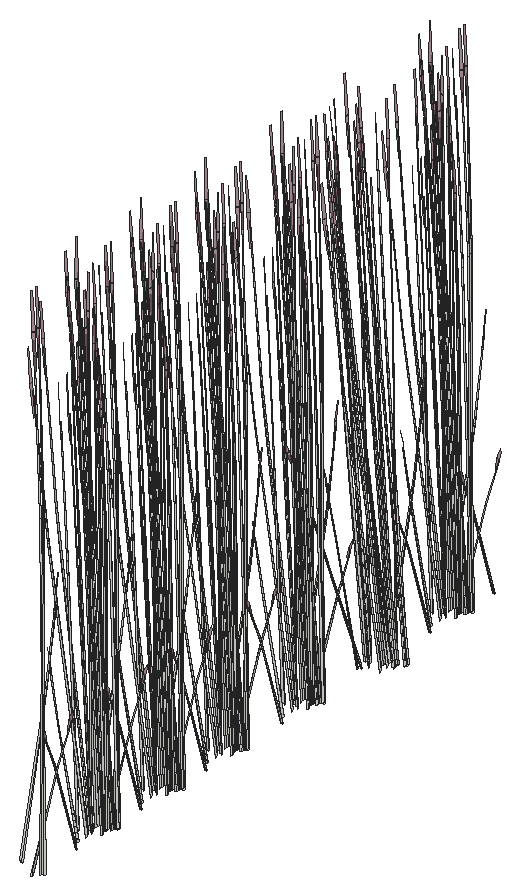
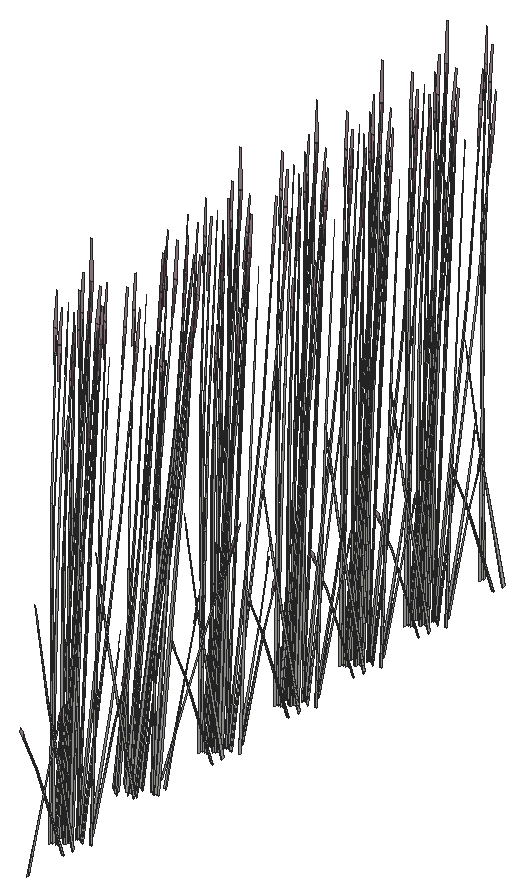
# SketchUp Ruby script. Lengths in inches.
U = 1.inch
M = Sketchup.active_model
def pt(a) = Geom::Point3d.new(a.map { |v| v * U })
def face(e, loops, mat)
  f = e.add_face(loops[0].map { |a| pt(a) })
  loops[1..].each { |l| e.add_face(l.map { |a| pt(a) }).erase! }
  f.material = f.back_material = mat if mat
  f
end
# faces: each face lists its corners as indices into pts; further lists are holes
def faces(e, pts, list, mat = nil) = list.each { |f| face(e, (f[0].is_a?(Array) ? f : [f]).map { |l| l.map { |i| pts[i] } }, mat) }
# xy, xz, yz: faces in a plane at the given z, y or x. An outline is a flat list of corners, or four numbers for a rectangle; further outlines are holes
def ring(l) = l.size == 4 ? [[l[0], l[1]], [l[2], l[1]], [l[2], l[3]], [l[0], l[3]]] : l.each_slice(2).to_a
def flat(e, list, mat, &to3) = list.each { |f| face(e, (f[0].is_a?(Array) ? f : [f]).map { |l| ring(l).map { |u, v| to3.(u, v) } }, mat) }
def xy(e, z, list, mat = nil) = flat(e, list, mat) { |x, y| [x, y, z] }
def xz(e, y, list, mat = nil) = flat(e, list, mat) { |x, z| [x, y, z] }
def yz(e, x, list, mat = nil) = flat(e, list, mat) { |y, z| [x, y, z] }
def lines(e, pts, list) = list.each { |a, b| e.add_line(pt(pts[a]), pt(pts[b])) }
# prism: a flat outline (further loops are holes) pulled along v
def prism(e, loops, v, mat = nil)
  f = face(e, loops, mat); d = Geom::Vector3d.new(v.map { |x| x * U })
  f.pushpull(f.normal.samedirection?(d) ? d.length : -d.length)
end
def box(e, o, s, mat = nil) = prism(e, [[o, [o[0] + s[0], o[1], o[2]], [o[0] + s[0], o[1] + s[1], o[2]], [o[0], o[1] + s[1], o[2]]]], [0, 0, s[2]], mat)
def at(x, y, z, deg = 0) = Geom::Transformation.translation(pt([x, y, z])) * Geom::Transformation.rotation(ORIGIN, Z_AXIS, deg.degrees)
def axes(o, x, y, z) = Geom::Transformation.new([*x, 0, *y, 0, *z, 0, *pt(o).to_a, 1])
def part(name) = M.definitions.add(name)
# library, detail: a bought-in or finely detailed component or shape, given as its bounding box
def library(name, o, s) = part(name).tap { |d| box(d.entities, o, s) }
def detail(e, o, s) = box(e.add_group.entities, o, s)
def put(e, d, t, mat = nil) = e.add_instance(d, t).tap { |i| i.material = mat if mat }
def group(e, t, mat = nil) = e.add_group.tap { |g| g.transformation = t; g.material = mat if mat }.entities
root = M.entities
M.materials.add("LightPink_Translucent").color = [144, 107, 117]
M.materials["LightPink_Translucent"].alpha = 0.75
c1 = part("blade")
p = [[2.15,0.21,22],[0,0.17,0],[0.09,0.45,0],[2.18,0.31,22],[2.29,0.31,22],[0.38,0.45,0],
  [2.48,0.24,33],[2.49,0.24,33],[2.48,0.22,33]]
faces(c1.entities,p,[[0,1,2,3],[4,5,2,3],[6,3,4,7],[8,0,3,6]])
c2 = part("seeds")
p = [[0.3,-0.1,1.38],[-0.01,-0.03,1.59],[-0.01,-0.03,0.03],[0.14,-0.07,-0.07],[0.29,-0.03,3],[0.15,0.01,3.11]]
faces(c2.entities,p,[[0,1,2,3],[1,0,4,5]],"LightPink_Translucent")
c3 = part("blade with seeds")
put(c3.entities,c1,at(0,0,0))
put(c3.entities,c2,axes([2.4,0.25,30.99],[1.5799,-0.05474,1.17369],[-0.12525,1.92788,0.29478],[-0.07173,-0.02425,1.56792]))
put(root,c3,axes([334.62,388.33,50.06],[0.63212,0.12701,0.27176],[-0.15814,0.45398,-0.32244],[-0.10462,0.05682,1.45692]))
put(root,c3,axes([335,388.57,50.1],[0.31568,0.39156,0],[-0.52815,0.21836,-0.456],[-0.12029,0.04973,1.44655]))
put(root,c3,axes([333.34,388.69,49.32],[0.08172,-0.02126,1.55816],[0.49154,0.11703,-0.23804],[0.01437,0.1319,0.26541]))
put(root,c3,axes([332.21,388.75,50.49],[0.45869,-0.0692,0.0575],[0.10545,0.27878,-0.76259],[-0.02908,0.14112,0.68355]))
put(root,c3,axes([333.7,394.53,49.32],[-0.08469,0.01408,1.55816],[-0.46834,-0.15847,-0.23804],[0.00786,-0.13218,0.26541]))
put(root,c3,axes([333,396.42,49.85],[-0.20736,-0.4007,-0.61707],[0.59731,-0.14431,-0.16195],[-0.02292,-0.13569,1.36206]))
put(root,c3,axes([333.61,394.8,49.88],[-0.34892,0.22417,-0.0344],[-0.3197,-0.24551,-0.15595],[-0.02251,-0.06957,0.51438]))
put(root,c3,axes([333.32,396.53,49.95],[0.24498,-0.3521,-0.39531],[0.50902,0.16945,0.19025],[0,-0.08116,1.26923]))
put(root,c3,axes([332.02,396.375,49.79],[0.35245,-0.2438,-0.27372],[0.35245,0.2438,0.27372],[0,-0.07853,1.22797]))
put(root,c3,axes([333.25,396.82,50.36],[-0.56863,-0.18645,-0.25709],[0.2738,-0.39352,-0.44182],[-0.01787,-0.09662,1.41118]))
put(root,c3,axes([333.42,396.58,50.09],[0.21952,0.43694,0.40429],[-0.62724,0.15194,0.15865],[0.00767,-0.08029,1.40366]))
put(root,c3,axes([333.31,396.93,50.4],[-0.24498,0.3521,0.39531],[-0.50902,-0.16945,-0.19025],[0,-0.08116,1.26923]))
put(root,c3,axes([334.36,396.97,50.03],[-0.46965,-0.33633,-0.05417],[0.46994,-0.33653,0],[-0.0164,-0.01174,1.55135]))
put(root,c3,axes([333.47,397.01,50.09],[0.63817,0.08233,0.40429],[-0.12987,0.46497,0.15865],[-0.09326,-0.0449,1.40366]))
put(root,c3,axes([333.13,397.75,50.1875],[0.54257,-0.10371,0.15589],[0.13397,0.38597,0.31002],[-0.04839,-0.05624,1.41735]))
put(root,c3,axes([333.94,397.66,49.95],[-0.16474,-0.33688,0],[0.47043,-0.11798,0],[0,0,1.36402]))
put(root,c3,axes([334.74,397.77,50.1875],[0.14586,-0.38834,0.15589],[0.53375,0.1099,0.31002],[-0.0922,0.00189,1.41735]))
put(root,c3,axes([333.83,397.82,49.94],[-0.50902,-0.17543,0],[0.24498,-0.36452,0],[0,0,1.43768]))
put(root,c3,axes([334.49,397.09,50.4],[0.54829,-0.02412,0.39531],[0.04958,0.40041,-0.19025],[-0.09816,0.04058,1.26923]))
put(root,c3,axes([334.61,398.21,49.9375],[-0.31175,-0.39292,-0.04544],[0.52815,-0.21836,0.456],[-0.13015,0.03741,1.44584]))
put(root,c3,axes([334.5,397.26,50.3125],[0.37303,0.23477,0.12794],[-0.31115,0.26487,-0.36534],[-0.08661,0.03581,1.11991]))
put(root,c3,axes([334.89,397.98,50.19],[0.47255,-0.19538,0.43871],[0.28245,0.35034,0],[-0.10763,0.0445,1.3917]))
put(root,c3,axes([334.46,398.16,49.79],[-0.47106,-0.09668,-0.27372],[0.11861,-0.34048,0.27372],[-0.09497,0.03926,1.22797]))
put(root,c3,axes([334.38,397.17,50.36],[0.05884,0.44587,-0.25709],[-0.6128,0.02696,-0.44182],[-0.10791,0.05939,1.41118]))
put(root,c3,axes([334.62,398.01,50.06],[0.63212,0.12701,0.27176],[-0.15814,0.45398,-0.32244],[-0.10462,0.05682,1.45692]))
put(root,c3,axes([335,398.25,50.1],[0.31568,0.39156,0],[-0.52815,0.21836,-0.456],[-0.12029,0.04973,1.44655]))
put(root,c3,axes([333.7,402.99,49.32],[-0.08469,0.01408,1.55816],[-0.46834,-0.15847,-0.23804],[0.00786,-0.13218,0.26541]))
put(root,c3,axes([333.34,398.375,49.32],[0.08172,-0.02126,1.55816],[0.49154,0.11703,-0.23804],[0.01437,0.1319,0.26541]))
put(root,c3,axes([332.21,398.43,50.49],[0.45869,-0.0692,0.0575],[0.10545,0.27878,-0.76259],[-0.02908,0.14112,0.68355]))
put(root,c3,axes([333,404.89,49.85],[-0.20736,-0.4007,-0.61707],[0.59731,-0.14431,-0.16195],[-0.02292,-0.13569,1.36206]))
put(root,c3,axes([333.61,403.26,49.88],[-0.34892,0.22417,-0.0344],[-0.3197,-0.24551,-0.15595],[-0.02251,-0.06957,0.51438]))
put(root,c3,axes([333.32,404.99,49.95],[0.24498,-0.3521,-0.39531],[0.50902,0.16945,0.19025],[0,-0.08116,1.26923]))
put(root,c3,axes([332.02,404.84,49.79],[0.35245,-0.2438,-0.27372],[0.35245,0.2438,0.27372],[0,-0.07853,1.22797]))
put(root,c3,axes([333.25,405.28,50.36],[-0.56863,-0.18645,-0.25709],[0.2738,-0.39352,-0.44182],[-0.01787,-0.09662,1.41118]))
put(root,c3,axes([333.42,405.04,50.09],[0.21952,0.43694,0.40429],[-0.62724,0.15194,0.15865],[0.00767,-0.08029,1.40366]))
put(root,c3,axes([333.31,405.39,50.4],[-0.24498,0.3521,0.39531],[-0.50902,-0.16945,-0.19025],[0,-0.08116,1.26923]))
put(root,c3,axes([334.36,405.43,50.03],[-0.46965,-0.33633,-0.05417],[0.46994,-0.33653,0],[-0.0164,-0.01174,1.55135]))
put(root,c3,axes([333.47,405.47,50.09],[0.63817,0.08233,0.40429],[-0.12987,0.46497,0.15865],[-0.09326,-0.0449,1.40366]))
put(root,c3,axes([333.13,406.21,50.1875],[0.54257,-0.10371,0.15589],[0.13397,0.38597,0.31002],[-0.04839,-0.05624,1.41735]))
put(root,c3,axes([333.94,406.125,49.95],[-0.16474,-0.33688,0],[0.47043,-0.11798,0],[0,0,1.36402]))
put(root,c3,axes([334.74,406.24,50.1875],[0.14586,-0.38834,0.15589],[0.53375,0.1099,0.31002],[-0.0922,0.00189,1.41735]))
put(root,c3,axes([333.83,406.28,49.94],[-0.50902,-0.17543,0],[0.24498,-0.36452,0],[0,0,1.43768]))
put(root,c3,axes([334.49,405.55,50.4],[0.54829,-0.02412,0.39531],[0.04958,0.40041,-0.19025],[-0.09816,0.04058,1.26923]))
put(root,c3,axes([334.61,406.67,49.9375],[-0.31175,-0.39292,-0.04544],[0.52815,-0.21836,0.456],[-0.13015,0.03741,1.44584]))
put(root,c3,axes([334.5,405.72,50.3125],[0.37303,0.23477,0.12794],[-0.31115,0.26487,-0.36534],[-0.08661,0.03581,1.11991]))
put(root,c3,axes([334.89,406.44,50.19],[0.47255,-0.19538,0.43871],[0.28245,0.35034,0],[-0.10763,0.0445,1.3917]))
put(root,c3,axes([334.46,406.62,49.79],[-0.47106,-0.09668,-0.27372],[0.11861,-0.34048,0.27372],[-0.09497,0.03926,1.22797]))
put(root,c3,axes([334.38,405.63,50.36],[0.05884,0.44587,-0.25709],[-0.6128,0.02696,-0.44182],[-0.10791,0.05939,1.41118]))
put(root,c3,axes([334.62,406.47,50.06],[0.63212,0.12701,0.27176],[-0.15814,0.45398,-0.32244],[-0.10462,0.05682,1.45692]))
put(root,c3,axes([335,406.72,50.1],[0.31568,0.39156,0],[-0.52815,0.21836,-0.456],[-0.12029,0.04973,1.44655]))
put(root,c3,axes([333.7,411.45,49.32],[-0.08469,0.01408,1.55816],[-0.46834,-0.15847,-0.23804],[0.00786,-0.13218,0.26541]))
put(root,c3,axes([333.34,406.83,49.32],[0.08172,-0.02126,1.55816],[0.49154,0.11703,-0.23804],[0.01437,0.1319,0.26541]))
put(root,c3,axes([332.21,406.89,50.49],[0.45869,-0.0692,0.0575],[0.10545,0.27878,-0.76259],[-0.02908,0.14112,0.68355]))
put(root,c3,axes([333,413.35,49.85],[-0.20736,-0.4007,-0.61707],[0.59731,-0.14431,-0.16195],[-0.02292,-0.13569,1.36206]))
put(root,c3,axes([333.61,411.73,49.88],[-0.34892,0.22417,-0.0344],[-0.3197,-0.24551,-0.15595],[-0.02251,-0.06957,0.51438]))
put(root,c3,axes([333.32,413.45,49.95],[0.24498,-0.3521,-0.39531],[0.50902,0.16945,0.19025],[0,-0.08116,1.26923]))
put(root,c3,axes([332.02,413.3,49.79],[0.35245,-0.2438,-0.27372],[0.35245,0.2438,0.27372],[0,-0.07853,1.22797]))
put(root,c3,axes([333.25,413.75,50.36],[-0.56863,-0.18645,-0.25709],[0.2738,-0.39352,-0.44182],[-0.01787,-0.09662,1.41118]))
put(root,c3,axes([333.42,413.51,50.09],[0.21952,0.43694,0.40429],[-0.62724,0.15194,0.15865],[0.00767,-0.08029,1.40366]))
put(root,c3,axes([333.31,413.85,50.4],[-0.24498,0.3521,0.39531],[-0.50902,-0.16945,-0.19025],[0,-0.08116,1.26923]))
put(root,c3,axes([334.36,413.9,50.03],[-0.46965,-0.33633,-0.05417],[0.46994,-0.33653,0],[-0.0164,-0.01174,1.55135]))
put(root,c3,axes([333.47,413.9375,50.09],[0.63817,0.08233,0.40429],[-0.12987,0.46497,0.15865],[-0.09326,-0.0449,1.40366]))
put(root,c3,axes([333.13,414.68,50.1875],[0.54257,-0.10371,0.15589],[0.13397,0.38597,0.31002],[-0.04839,-0.05624,1.41735]))
put(root,c3,axes([333.94,414.59,49.95],[-0.16474,-0.33688,0],[0.47043,-0.11798,0],[0,0,1.36402]))
put(root,c3,axes([334.74,414.7,50.1875],[0.14586,-0.38834,0.15589],[0.53375,0.1099,0.31002],[-0.0922,0.00189,1.41735]))
put(root,c3,axes([333.83,414.74,49.94],[-0.50902,-0.17543,0],[0.24498,-0.36452,0],[0,0,1.43768]))
put(root,c3,axes([334.49,414.01,50.4],[0.54829,-0.02412,0.39531],[0.04958,0.40041,-0.19025],[-0.09816,0.04058,1.26923]))
put(root,c3,axes([334.61,415.14,49.9375],[-0.31175,-0.39292,-0.04544],[0.52815,-0.21836,0.456],[-0.13015,0.03741,1.44584]))
put(root,c3,axes([334.5,414.1875,50.3125],[0.37303,0.23477,0.12794],[-0.31115,0.26487,-0.36534],[-0.08661,0.03581,1.11991]))
put(root,c3,axes([334.89,414.91,50.19],[0.47255,-0.19538,0.43871],[0.28245,0.35034,0],[-0.10763,0.0445,1.3917]))
put(root,c3,axes([334.46,415.09,49.79],[-0.47106,-0.09668,-0.27372],[0.11861,-0.34048,0.27372],[-0.09497,0.03926,1.22797]))
put(root,c3,axes([334.38,414.1,50.36],[0.05884,0.44587,-0.25709],[-0.6128,0.02696,-0.44182],[-0.10791,0.05939,1.41118]))
put(root,c3,axes([334.62,414.9375,50.06],[0.63212,0.12701,0.27176],[-0.15814,0.45398,-0.32244],[-0.10462,0.05682,1.45692]))
put(root,c3,axes([335,415.18,50.1],[0.31568,0.39156,0],[-0.52815,0.21836,-0.456],[-0.12029,0.04973,1.44655]))
put(root,c3,axes([333.34,415.3,49.32],[0.08172,-0.02126,1.55816],[0.49154,0.11703,-0.23804],[0.01437,0.1319,0.26541]))
put(root,c3,axes([332.21,415.35,50.49],[0.45869,-0.0692,0.0575],[0.10545,0.27878,-0.76259],[-0.02908,0.14112,0.68355]))
put(root,c3,axes([333.7,421.35,49.32],[-0.08469,0.01408,1.55816],[-0.46834,-0.15847,-0.23804],[0.00786,-0.13218,0.26541]))
put(root,c3,axes([333,423.25,49.85],[-0.20736,-0.4007,-0.61707],[0.59731,-0.14431,-0.16195],[-0.02292,-0.13569,1.36206]))
put(root,c3,axes([333.61,421.625,49.88],[-0.34892,0.22417,-0.0344],[-0.3197,-0.24551,-0.15595],[-0.02251,-0.06957,0.51438]))
put(root,c3,axes([333.32,423.35,49.95],[0.24498,-0.3521,-0.39531],[0.50902,0.16945,0.19025],[0,-0.08116,1.26923]))
put(root,c3,axes([332.02,423.2,49.79],[0.35245,-0.2438,-0.27372],[0.35245,0.2438,0.27372],[0,-0.07853,1.22797]))
put(root,c3,axes([333.25,423.65,50.36],[-0.56863,-0.18645,-0.25709],[0.2738,-0.39352,-0.44182],[-0.01787,-0.09662,1.41118]))
put(root,c3,axes([333.42,423.41,50.09],[0.21952,0.43694,0.40429],[-0.62724,0.15194,0.15865],[0.00767,-0.08029,1.40366]))
put(root,c3,axes([333.31,423.75,50.4],[-0.24498,0.3521,0.39531],[-0.50902,-0.16945,-0.19025],[0,-0.08116,1.26923]))
put(root,c3,axes([334.36,423.8,50.03],[-0.46965,-0.33633,-0.05417],[0.46994,-0.33653,0],[-0.0164,-0.01174,1.55135]))
put(root,c3,axes([333.47,423.84,50.09],[0.63817,0.08233,0.40429],[-0.12987,0.46497,0.15865],[-0.09326,-0.0449,1.40366]))
put(root,c3,axes([333.13,424.58,50.1875],[0.54257,-0.10371,0.15589],[0.13397,0.38597,0.31002],[-0.04839,-0.05624,1.41735]))
put(root,c3,axes([333.94,424.49,49.95],[-0.16474,-0.33688,0],[0.47043,-0.11798,0],[0,0,1.36402]))
put(root,c3,axes([334.74,424.6,50.1875],[0.14586,-0.38834,0.15589],[0.53375,0.1099,0.31002],[-0.0922,0.00189,1.41735]))
put(root,c3,axes([333.83,424.64,49.94],[-0.50902,-0.17543,0],[0.24498,-0.36452,0],[0,0,1.43768]))
put(root,c3,axes([334.49,423.91,50.4],[0.54829,-0.02412,0.39531],[0.04958,0.40041,-0.19025],[-0.09816,0.04058,1.26923]))
put(root,c3,axes([334.61,425.04,49.9375],[-0.31175,-0.39292,-0.04544],[0.52815,-0.21836,0.456],[-0.13015,0.03741,1.44584]))
put(root,c3,axes([334.5,424.08,50.3125],[0.37303,0.23477,0.12794],[-0.31115,0.26487,-0.36534],[-0.08661,0.03581,1.11991]))
put(root,c3,axes([334.89,424.81,50.19],[0.47255,-0.19538,0.43871],[0.28245,0.35034,0],[-0.10763,0.0445,1.3917]))
put(root,c3,axes([334.46,424.99,49.79],[-0.47106,-0.09668,-0.27372],[0.11861,-0.34048,0.27372],[-0.09497,0.03926,1.22797]))
put(root,c3,axes([334.38,424,50.36],[0.05884,0.44587,-0.25709],[-0.6128,0.02696,-0.44182],[-0.10791,0.05939,1.41118]))
put(root,c3,axes([334.62,424.83,50.06],[0.63212,0.12701,0.27176],[-0.15814,0.45398,-0.32244],[-0.10462,0.05682,1.45692]))
put(root,c3,axes([335,425.08,50.1],[0.31568,0.39156,0],[-0.52815,0.21836,-0.456],[-0.12029,0.04973,1.44655]))
put(root,c3,axes([333.34,425.2,49.32],[0.08172,-0.02126,1.55816],[0.49154,0.11703,-0.23804],[0.01437,0.1319,0.26541]))
put(root,c3,axes([332.21,425.25,50.49],[0.45869,-0.0692,0.0575],[0.10545,0.27878,-0.76259],[-0.02908,0.14112,0.68355]))
put(root,c3,axes([334.13,431.15,50.29],[-0.03058,0.12783,1.26356],[-0.44698,0.10701,-0.27174],[-0.10448,-0.16522,0.54024]))
put(root,c3,axes([334.59,432.77,49.85],[-0.20736,-0.4007,-0.61707],[0.59731,-0.14431,-0.16195],[-0.02292,-0.13569,1.36206]))
put(root,c3,axes([333.36,432.71,49.78],[0,-0.39075,-0.43871],[0.56491,0,0],[0,-0.089,1.3917]))
put(root,c3,axes([333.46,431.55,49.88],[-0.14565,0.31907,-0.0344],[-0.44829,-0.09815,-0.15595],[-0.06806,-0.05219,0.51438]))
put(root,c3,axes([334.84,433.16,50.36],[-0.56863,-0.18645,-0.25709],[0.2738,-0.39352,-0.44182],[-0.01787,-0.09662,1.41118]))
put(root,c3,axes([333.22,433.01,50.1],[-0.63136,0,0],[0,-0.43672,-0.456],[0,-0.09947,1.44655]))
put(root,c3,axes([333.71,432.89,50.06],[-0.46965,0.32852,0.27176],[-0.46994,-0.32506,-0.32244],[-0.0164,-0.09329,1.45692]))
put(root,c3,axes([334.98,433.58,50.16],[0.13383,-0.46302,-0.20702],[0.63453,0.08071,0.45303],[-0.11087,-0.06394,1.38231]))
put(root,c3,axes([333.61,433.07,50.19],[0,0.39075,0.43871],[-0.56491,0,0],[0,-0.089,1.3917]))
put(root,c3,axes([334.94,433.39,49.95],[-0.30332,-0.32798,-0.39531],[0.45944,-0.23096,0.19025],[-0.09816,-0.04058,1.26923]))
put(root,c3,axes([334.11,434.12,49.79],[-0.11861,-0.34048,-0.27372],[0.47106,-0.09668,0.27372],[-0.09497,-0.03926,1.22797]))
put(root,c3,axes([335.26,433.57,50.36],[-0.50979,0.25942,-0.25709],[-0.339,-0.36656,-0.44182],[-0.12578,-0.03723,1.41118]))
put(root,c3,axes([335.22,433.6875,50.3125],[-0.09741,0.34873,0.12794],[-0.4759,-0.06053,-0.36534],[-0.08661,-0.03581,1.11991]))
put(root,c3,axes([335.84,433.69,50.18],[-0.49304,-0.31451,-0.2226],[0.41487,-0.35316,0.48713],[-0.13277,0.03679,1.48635]))
put(root,c3,axes([334.54,434.29,50.19],[0.47255,0.19538,0.43871],[-0.28245,0.35034,0],[-0.10763,-0.0445,1.3917]))
put(root,c3,axes([335.59,433.625,49.95],[-0.54829,0.02412,-0.39531],[-0.04958,-0.40041,0.19025],[-0.09816,0.04058,1.26923]))
put(root,c3,axes([336.19,434.55,49.9375],[-0.31175,-0.39292,-0.04544],[0.52815,-0.21836,0.456],[-0.13015,0.03741,1.44584]))
put(root,c3,axes([336.05,434.5,49.79],[-0.47106,-0.09668,-0.27372],[0.11861,-0.34048,0.27372],[-0.09497,0.03926,1.22797]))
put(root,c3,axes([335.97,433.52,50.36],[0.05884,0.44587,-0.25709],[-0.6128,0.02696,-0.44182],[-0.10791,0.05939,1.41118]))
put(root,c3,axes([335.6,433.86,49.82],[-0.34009,0.2937,-0.55095],[-0.42248,-0.26632,-0.1446],[-0.13628,0.07327,1.21613]))
put(root,c3,axes([336.16,434.66,49.78],[-0.47255,0.19538,-0.43871],[-0.28245,-0.35034,0],[-0.10763,0.0445,1.3917]))
put(root,c3,axes([333.8,434.77,50.49],[0.45869,-0.0692,0.0575],[0.10545,0.27878,-0.76259],[-0.02908,0.14112,0.68355]))
put(root,c3,axes([333.7,440.74,49.32],[-0.08469,0.01408,1.55816],[-0.46834,-0.15847,-0.23804],[0.00786,-0.13218,0.26541]))
put(root,c3,axes([333,442.63,49.85],[-0.20736,-0.4007,-0.61707],[0.59731,-0.14431,-0.16195],[-0.02292,-0.13569,1.36206]))
put(root,c3,axes([333.61,441.01,49.88],[-0.34892,0.22417,-0.0344],[-0.3197,-0.24551,-0.15595],[-0.02251,-0.06957,0.51438]))
put(root,c3,axes([333.32,442.74,49.95],[0.24498,-0.3521,-0.39531],[0.50902,0.16945,0.19025],[0,-0.08116,1.26923]))
put(root,c3,axes([332.02,442.59,49.79],[0.35245,-0.2438,-0.27372],[0.35245,0.2438,0.27372],[0,-0.07853,1.22797]))
put(root,c3,axes([333.25,443.03,50.36],[-0.56863,-0.18645,-0.25709],[0.2738,-0.39352,-0.44182],[-0.01787,-0.09662,1.41118]))
put(root,c3,axes([332.02,442.94,50.19],[0,0.39075,0.43871],[-0.56491,0,0],[0,-0.089,1.3917]))
put(root,c3,axes([333.42,442.79,50.09],[0.21952,0.43694,0.40429],[-0.62724,0.15194,0.15865],[0.00767,-0.08029,1.40366]))
put(root,c3,axes([333.31,443.14,50.4],[-0.24498,0.3521,0.39531],[-0.50902,-0.16945,-0.19025],[0,-0.08116,1.26923]))
put(root,c3,axes([334.36,443.18,50.03],[-0.46965,-0.33633,-0.05417],[0.46994,-0.33653,0],[-0.0164,-0.01174,1.55135]))
put(root,c3,axes([333.47,443.22,50.09],[0.63817,0.08233,0.40429],[-0.12987,0.46497,0.15865],[-0.09326,-0.0449,1.40366]))
put(root,c3,axes([333.13,443.96,50.1875],[0.54257,-0.10371,0.15589],[0.13397,0.38597,0.31002],[-0.04839,-0.05624,1.41735]))
put(root,c3,axes([333.94,443.875,49.95],[-0.16474,-0.33688,0],[0.47043,-0.11798,0],[0,0,1.36402]))
put(root,c3,axes([334.74,443.99,50.1875],[0.14586,-0.38834,0.15589],[0.53375,0.1099,0.31002],[-0.0922,0.00189,1.41735]))
put(root,c3,axes([333.83,444.03,49.94],[-0.50902,-0.17543,0],[0.24498,-0.36452,0],[0,0,1.43768]))
put(root,c3,axes([334.49,443.3,50.4],[0.54829,-0.02412,0.39531],[0.04958,0.40041,-0.19025],[-0.09816,0.04058,1.26923]))
put(root,c3,axes([334.61,444.42,49.9375],[-0.31175,-0.39292,-0.04544],[0.52815,-0.21836,0.456],[-0.13015,0.03741,1.44584]))
put(root,c3,axes([334.5,443.47,50.3125],[0.37303,0.23477,0.12794],[-0.31115,0.26487,-0.36534],[-0.08661,0.03581,1.11991]))
put(root,c3,axes([334.89,444.19,50.19],[0.47255,-0.19538,0.43871],[0.28245,0.35034,0],[-0.10763,0.0445,1.3917]))
put(root,c3,axes([334.46,444.37,49.79],[-0.47106,-0.09668,-0.27372],[0.11861,-0.34048,0.27372],[-0.09497,0.03926,1.22797]))
put(root,c3,axes([334.38,443.38,50.36],[0.05884,0.44587,-0.25709],[-0.6128,0.02696,-0.44182],[-0.10791,0.05939,1.41118]))
put(root,c3,axes([334.62,444.22,50.06],[0.63212,0.12701,0.27176],[-0.15814,0.45398,-0.32244],[-0.10462,0.05682,1.45692]))
put(root,c3,axes([335,444.46,50.1],[0.31568,0.39156,0],[-0.52815,0.21836,-0.456],[-0.12029,0.04973,1.44655]))
put(root,c3,axes([333.7,449.11,49.32],[-0.08469,0.01408,1.55816],[-0.46834,-0.15847,-0.23804],[0.00786,-0.13218,0.26541]))
put(root,c3,axes([333.34,444.58,49.32],[0.08172,-0.02126,1.55816],[0.49154,0.11703,-0.23804],[0.01437,0.1319,0.26541]))
put(root,c3,axes([332.21,444.64,50.49],[0.45869,-0.0692,0.0575],[0.10545,0.27878,-0.76259],[-0.02908,0.14112,0.68355]))
